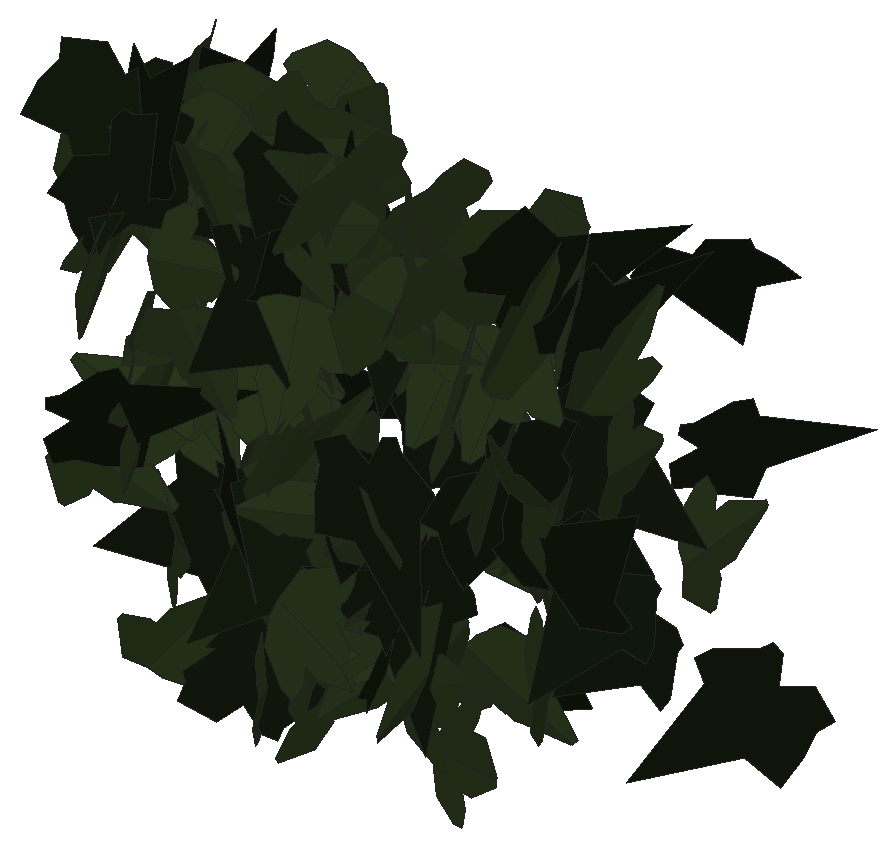
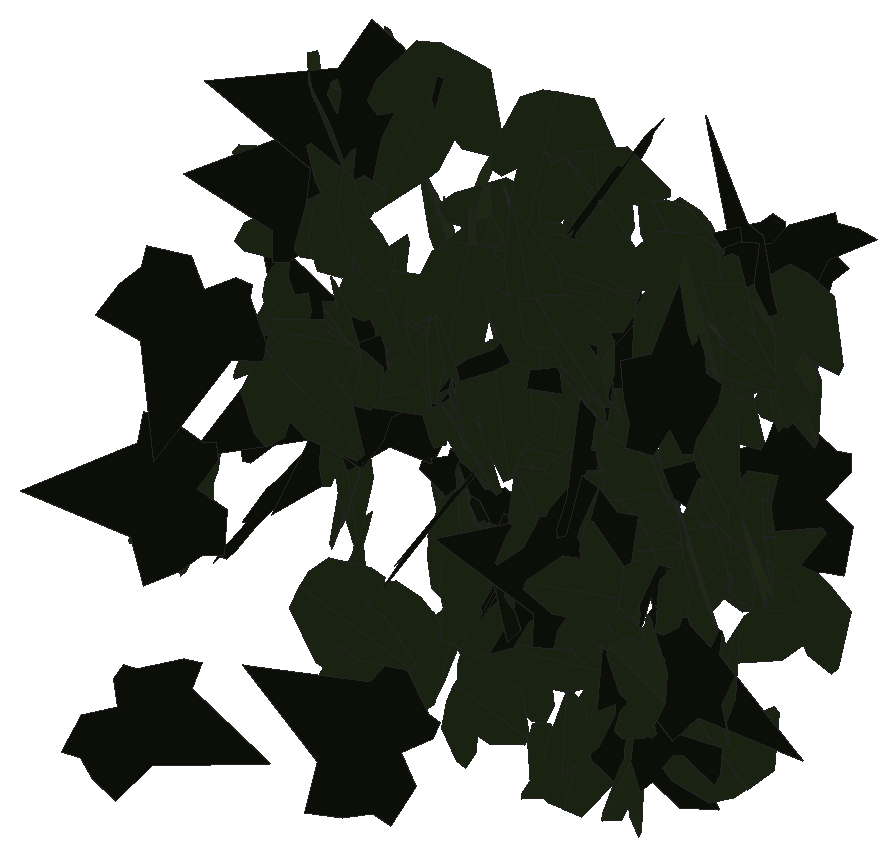
# SketchUp Ruby script. Lengths in inches.
U = 1.inch
M = Sketchup.active_model
def pt(a) = Geom::Point3d.new(a.map { |v| v * U })
def face(e, loops, mat)
  f = e.add_face(loops[0].map { |a| pt(a) })
  loops[1..].each { |l| e.add_face(l.map { |a| pt(a) }).erase! }
  f.material = f.back_material = mat if mat
  f
end
# faces: each face lists its corners as indices into pts; further lists are holes
def faces(e, pts, list, mat = nil) = list.each { |f| face(e, (f[0].is_a?(Array) ? f : [f]).map { |l| l.map { |i| pts[i] } }, mat) }
# xy, xz, yz: faces in a plane at the given z, y or x. An outline is a flat list of corners, or four numbers for a rectangle; further outlines are holes
def ring(l) = l.size == 4 ? [[l[0], l[1]], [l[2], l[1]], [l[2], l[3]], [l[0], l[3]]] : l.each_slice(2).to_a
def flat(e, list, mat, &to3) = list.each { |f| face(e, (f[0].is_a?(Array) ? f : [f]).map { |l| ring(l).map { |u, v| to3.(u, v) } }, mat) }
def xy(e, z, list, mat = nil) = flat(e, list, mat) { |x, y| [x, y, z] }
def xz(e, y, list, mat = nil) = flat(e, list, mat) { |x, z| [x, y, z] }
def yz(e, x, list, mat = nil) = flat(e, list, mat) { |y, z| [x, y, z] }
def lines(e, pts, list) = list.each { |a, b| e.add_line(pt(pts[a]), pt(pts[b])) }
# prism: a flat outline (further loops are holes) pulled along v
def prism(e, loops, v, mat = nil)
  f = face(e, loops, mat); d = Geom::Vector3d.new(v.map { |x| x * U })
  f.pushpull(f.normal.samedirection?(d) ? d.length : -d.length)
end
def box(e, o, s, mat = nil) = prism(e, [[o, [o[0] + s[0], o[1], o[2]], [o[0] + s[0], o[1] + s[1], o[2]], [o[0], o[1] + s[1], o[2]]]], [0, 0, s[2]], mat)
def at(x, y, z, deg = 0) = Geom::Transformation.translation(pt([x, y, z])) * Geom::Transformation.rotation(ORIGIN, Z_AXIS, deg.degrees)
def axes(o, x, y, z) = Geom::Transformation.new([*x, 0, *y, 0, *z, 0, *pt(o).to_a, 1])
def part(name) = M.definitions.add(name)
# library, detail: a bought-in or finely detailed component or shape, given as its bounding box
def library(name, o, s) = part(name).tap { |d| box(d.entities, o, s) }
def detail(e, o, s) = box(e.add_group.entities, o, s)
def put(e, d, t, mat = nil) = e.add_instance(d, t).tap { |i| i.material = mat if mat }
def group(e, t, mat = nil) = e.add_group.tap { |g| g.transformation = t; g.material = mat if mat }.entities
root = M.entities
M.materials.add("efeu1").color = [18, 25, 13]
M.materials.add("efeu2").color = [43, 57, 29]
c1 = part("ivyleaf_10")
p = [[0,0.5,-0.03],[-0.0625,2.02,-0.43],[-0.19,2.01,-0.46],[-0.54,1.05,-0.29],[-0.52,0.625,-0.18],[-0.83,0.76,-0.28],
  [-1.16,0.64,-0.33],[-1.15,0.33,-0.24],[-0.77,-0.39,0.02],[-0.3,-0.51,0.16],[0.04,-0.48,0.23],[-0.02,2.01,-0.4375],
  [-0.06,2.01,-0.43],[0.04,-0.49,0.23],[0.67,-0.49,0.14],[1.38,0.36,-0.2],[1.375,0.51,-0.24],[0.81,0.65,-0.19],
  [0.62,0.59,-0.15],[0.6,1.09,-0.28],[0.5,1.23,-0.31]]
faces(c1.entities,p,[[0,1,2,3,4,5,6,7,8,9,10],[11,12,0,13,14,15,16,17,18,19,20]],"efeu2")
c2 = part("ivyleaf_9")
p = [[1.54,2.16,1.25],[1.36,2.04,1.19],[-0.21,0.99,0.68],[-0.71,1.11,0.82],[-0.85,0.86,0.67],[-0.8,0.17,0.21],
  [-0.9,-0.01,0.1],[-0.67,-0.16,-0.02],[-0.08,-0.08,-0.05],[-0.03,-0.6,-0.4],[0.65,-0.88,-0.66],[0.83,-0.6,-0.49],
  [1.29,-0.42,-0.43],[1.8125,-0.07,-0.26],[1.21,0.44,0.15]]
faces(c2.entities,p,[[0,1,2,3,4,5,6,7,8,9,10,11,12,13,14]],"efeu1")
put(root,c1,axes([531.59,135.63,168.51],[-0.39651,0.03608,0.65448],[0.62652,-0.20395,0.39082],[0.19265,0.73754,0.07605]))
put(root,c1,axes([530.57,135.38,169.3],[0.4498,-0.67197,0.0682],[-0.028,0.06332,0.80854],[-0.67485,-0.45052,0.01191]))
put(root,c1,axes([524.71,135.68,170.1875],[0.13317,-0.67555,0.22901],[0.09772,-0.21349,-0.6866],[0.70659,0.15685,0.0518]))
put(root,c1,axes([529.39,135.33,167.53],[-0.4084,0.02461,0.55664],[-0.55643,0.01796,-0.40903],[-0.02905,-0.69016,0.00921]))
put(root,c2,axes([529.11,135.65,168.17],[0.29259,-0.81264,-0.10232],[-0.03731,0.09532,-0.8637],[0.81821,0.29495,-0.00279]))
put(root,c2,axes([524.8,134.97,167.72],[0.24324,0.53868,-0.57318],[0.23052,0.52479,0.59104],[0.75204,-0.3351,0.00422]))
put(root,c1,axes([528.37,135.0625,165.95],[-0.00344,0.62956,0.46716],[-0.00301,0.46715,-0.62957],[-0.78395,-0.00456,0.00037]))
put(root,c1,axes([528.69,135.78,167.27],[0.00736,0.01589,0.74245],[-0.5731,-0.47205,0.01578],[0.47226,-0.5731,0.00758]))
put(root,c1,axes([530.04,136.0625,165.72],[0.07231,-0.35282,0.70235],[0.17205,-0.6811,-0.35986],[0.76692,0.18606,0.01451]))
put(root,c2,axes([527.125,136.19,169.88],[-0.17709,-0.46496,0.63976],[-0.14722,-0.62476,-0.49481],[0.77705,-0.22433,0.05205]))
put(root,c1,axes([529.74,135.83,165.03],[0.32065,-0.23828,-0.71476],[0.54937,-0.45766,0.39903],[-0.51561,-0.6358,-0.01935]))
put(root,c2,axes([526.64,136.1,166.29],[-0.15856,0.00295,0.8534],[0.08395,-0.86374,0.01858],[0.84927,0.08593,0.15749]))
put(root,c1,axes([531.75,135.19,170.95],[0.26182,-0.59476,0.61403],[-0.20768,0.57869,0.64909],[-0.82924,-0.33272,0.03131]))
put(root,c1,axes([525.67,135.77,170.07],[0.14569,-0.08799,-0.68476],[0.61926,-0.29273,0.16937],[-0.30521,-0.63595,0.01678]))
put(root,c1,axes([530.76,135.37,172.03],[-0.34024,-0.63647,-0.55717],[0.23635,0.50511,-0.72132],[0.8122,-0.41361,-0.0235]))
put(root,c1,axes([527.8,135.91,171.3],[0.23201,-0.23226,-0.7183],[0.65895,-0.30437,0.31126],[-0.36836,-0.69076,0.10437]))
put(root,c2,axes([527.66,136.26,166.49],[-0.52969,-0.47413,0.28475],[-0.20039,-0.20296,-0.71071],[0.51549,-0.56609,0.01632]))
put(root,c1,axes([526.08,135.67,169.24],[-0.68378,-0.15233,-0.18445],[0.1801,0.0398,-0.70054],[0.15744,-0.7071,0.0003]))
put(root,c2,axes([532.01,135.89,167.36],[-0.21716,-0.06392,0.76179],[0.64532,-0.4399,0.14705],[0.40984,0.65877,0.17211]))
put(root,c1,axes([524.65,135.6,169.89],[0.27816,-0.66408,0.30344],[-0.0927,0.28996,0.71957],[-0.72421,-0.29218,0.02444]))
put(root,c1,axes([525.15,136.08,167.83],[0.14834,-0.6526,0.26133],[0.10541,-0.24342,-0.6677],[0.69503,0.1762,0.04549]))
put(root,c1,axes([527.63,135.86,169.73],[0.70962,0.20851,-0.02329],[-0.02405,-0.00075,-0.7396],[-0.20842,0.71,0.00606]))
put(root,c2,axes([525,135.44,171.52],[0.0496,-0.18551,-0.74559],[0.02226,0.74717,-0.18442],[0.76799,-0.00968,0.0535]))
put(root,c2,axes([524.53,136.2,172.16],[-0.29661,-0.7166,-0.13537],[0.06053,0.12144,-0.7755],[0.72676,-0.30258,0.00934]))
put(root,c2,axes([525.02,136.02,171.38],[-0.22619,0.33505,0.65354],[0.26485,-0.60061,0.39958],[0.685,0.34285,0.06131]))
put(root,c2,axes([529.45,136.08,166.65],[-0.50927,-0.22396,-0.63282],[0.58838,0.23345,-0.55613],[0.32314,-0.77802,0.01529]))
put(root,c1,axes([529.29,136.21,165.14],[-0.29206,-0.33727,0.57779],[-0.38365,-0.43207,-0.44612],[0.5481,-0.48214,-0.00439]))
put(root,c1,axes([530.93,135.99,168.77],[0.18073,-0.72055,-0.03775],[-0.00782,0.03696,-0.74287],[0.7215,0.1809,0.0014]))
put(root,c1,axes([526.12,135.89,171.53],[-0.61442,0.2705,-0.22588],[0.20711,-0.09015,-0.67132],[-0.28512,-0.64838,-0.0009]))
put(root,c1,axes([528.6,135.74,172.3],[-0.25568,-0.77369,-0.37196],[0.10203,0.35797,-0.81472],[0.85237,-0.27493,-0.01405]))
put(root,c2,axes([527.33,135.93,172.1875],[0.40346,-0.57241,-0.32294],[-0.16635,0.27766,-0.69997],[0.63583,0.43586,0.02179]))
put(root,c1,axes([527.67,136.01,172.01],[-0.50904,-0.44696,0.07923],[-0.05516,-0.05725,-0.67738],[0.45056,-0.51197,0.00658]))
put(root,c1,axes([524.51,135.91,171.24],[-0.76025,-0.05515,-0.26231],[0.26294,-0.00024,-0.76203],[0.05205,-0.80423,0.01821]))
put(root,c1,axes([524.29,135.81,166.73],[-0.40222,-0.21698,-0.51948],[0.48379,0.19327,-0.45532],[0.28789,-0.62793,0.03937]))
put(root,c1,axes([529.18,135.76,170.67],[-0.39801,-0.32731,-0.64646],[0.55624,0.33466,-0.51191],[0.46437,-0.68141,0.0591]))
put(root,c1,axes([528.95,136.02,165.72],[0.47088,0.11639,0.50683],[0.47941,0.16773,-0.48393],[-0.20147,0.67117,0.03305]))
put(root,c1,axes([525.4,136,163.95],[-0.38309,-0.40564,0.35463],[0.25571,0.24613,0.55776],[-0.47425,0.46037,0.01427]))
put(root,c1,axes([529.36,136.25,165.5],[0.36558,-0.67525,-0.10081],[0.05545,-0.08461,0.76781],[-0.68047,-0.36967,0.00841]))
put(root,c1,axes([528.4375,136.04,165.69],[0.66506,0.16037,-0.13782],[0.13359,0.03394,0.68412],[0.16392,-0.67834,0.00164]))
put(root,c1,axes([527.77,135.76,167.48],[0.09933,-0.44647,0.64173],[-0.08257,0.63728,0.45615],[-0.77739,-0.12473,0.03355]))
put(root,c2,axes([532.29,136.82,167.18],[-0.28597,-0.62776,0.33162],[-0.13912,-0.30103,-0.68983],[0.69621,-0.31801,-0.00163]))
put(root,c1,axes([525.04,136.43,167.14],[0.27394,0.3777,0.53924],[-0.41946,-0.35004,0.45827],[0.50744,-0.49325,0.0877]))
put(root,c1,axes([526.21,136.3,171.96],[0.64179,-0.18739,-0.23723],[-0.22442,0.07766,-0.6685],[0.20255,0.67981,0.01098]))
put(root,c1,axes([531.85,136.53,171.9],[0.54873,-0.47539,0.28764],[0.21523,-0.19085,-0.726],[0.51226,0.58942,-0.00308]))
put(root,c1,axes([525.02,136.57,165.31],[-0.21851,0.12823,0.66954],[0.59328,-0.31054,0.2531],[0.33578,0.63214,-0.01148]))
put(root,c2,axes([527.3,136.54,169.68],[0.4162,0.40639,0.59318],[-0.44093,-0.39714,0.58146],[0.56797,-0.60611,0.01673]))
put(root,c1,axes([528.16,136.59,170.39],[0.24682,-0.40499,-0.55279],[0.39299,-0.39768,0.46682],[-0.56139,-0.45645,0.08375]))
put(root,c1,axes([527.43,135.84,167.23],[0.06635,-0.43948,0.72964],[-0.03839,0.72956,0.44293],[-0.85091,-0.06718,0.03691]))
put(root,c2,axes([529.33,135.88,165.74],[-0.4637,0.24143,-0.6951],[-0.64038,0.27227,0.52177],[0.36243,0.78996,0.0326]))
put(root,c2,axes([526.49,136.31,163.57],[-0.59702,0.09361,0.49924],[0.45949,-0.22888,0.59239],[0.21652,0.74384,0.11945]))
put(root,c1,axes([530.2,135.98,164.11],[-0.13059,0.40394,0.56917],[-0.22728,0.52288,-0.42323],[-0.6599,-0.26002,0.03313]))
put(root,c2,axes([531.18,136.05,171.41],[0.20779,0.0048,0.83066],[0.79376,0.25127,-0.20002],[-0.24488,0.81856,0.05653]))
put(root,c1,axes([527.65,136.875,167.11],[-0.12673,-0.53979,-0.46269],[-0.12428,-0.44593,0.55427],[-0.70001,0.17689,-0.01464]))
put(root,c1,axes([526.96,136.34,164.96],[-0.43065,0.32413,-0.49227],[-0.4355,0.23582,0.53626],[0.39715,0.61006,0.05426]))
put(root,c1,axes([527.15,136.58,169.78],[-0.42261,0.38138,-0.38604],[0.29375,-0.25063,-0.56919],[-0.45628,-0.5146,-0.00888]))
put(root,c1,axes([527.43,136.9,163.45],[-0.13135,-0.56196,-0.43447],[-0.11411,-0.41941,0.57697],[-0.7011,0.17354,-0.0125]))
put(root,c1,axes([529.17,136.53,170.8125],[0.28881,-0.68795,-0.15673],[-0.06917,0.14093,-0.74606],[0.70218,0.29684,-0.00903]))
put(root,c1,axes([529.06,137.07,165.72],[-0.016,0.00559,-0.7466],[-0.29074,-0.68787,0.00108],[-0.68769,0.29069,0.01691]))
put(root,c1,axes([524.93,136.84,171.14],[0.11394,-0.43975,-0.5067],[0.35842,-0.39457,0.42303],[-0.56714,-0.33771,0.16555]))
put(root,c1,axes([529.65,136.08,170.66],[-0.20672,0.40739,-0.74788],[-0.39152,0.63798,0.45575],[0.7563,0.44162,0.03152]))
put(root,c2,axes([528.29,136.24,165.95],[0.64479,0.3981,-0.16174],[-0.14511,-0.07279,-0.75766],[-0.40446,0.66077,0.01398]))
put(root,c1,axes([524.32,136.89,168.23],[0.35167,-0.49671,0.35568],[0.24419,-0.2619,-0.60719],[0.56,0.42613,0.04141]))
put(root,c2,axes([525.94,136.77,165.85],[-0.08076,-0.06061,-0.80323],[-0.65452,-0.4656,0.10094],[-0.46952,0.65947,-0.00256]))
put(root,c1,axes([527.71,137.19,165.3],[-0.12104,-0.29918,0.64305],[0.00431,-0.65265,-0.30283],[0.70923,-0.04709,0.11158]))
put(root,c1,axes([528.6,137.24,164.95],[-0.02881,-0.12579,0.72322],[0.1565,-0.70819,-0.11695],[0.7172,0.14948,0.05457]))
put(root,c2,axes([528.02,136.55,167.23],[0.50992,-0.52739,-0.44858],[-0.29596,0.33762,-0.73336],[0.62593,0.58929,0.0187]))
put(root,c1,axes([527.48,137.09,166.63],[-0.26848,0.27606,0.61112],[0.39362,-0.46807,0.38436],[0.5429,0.47588,0.02354]))
put(root,c1,axes([532.24,136.57,170.12],[0.02248,-0.6388,0.40227],[-0.02157,0.40174,0.63916],[-0.7546,-0.03051,-0.00629]))
put(root,c1,axes([524.96,136.74,167.33],[0.73535,-0.13555,-0.05695],[0.05617,-0.00943,0.74774],[-0.13588,-0.73749,0.0009]))
put(root,c1,axes([530.39,136.91,169.71],[0.73234,0.08478,-0.17386],[-0.17379,-0.01055,-0.73718],[-0.08493,0.75262,0.00925]))
put(root,c1,axes([531.0625,136.76,166.97],[-0.46824,0.5948,-0.09438],[0.0586,-0.07399,-0.75699],[-0.59938,-0.4719,-0.00027]))
put(root,c1,axes([526.71,136.38,163.76],[0,-0.08958,-0.67894],[-0.10214,0.67135,-0.08858],[0.67717,0.10126,-0.01336]))
put(root,c1,axes([524.82,136.46,167.79],[0.0479,0.03506,0.74705],[0.4376,0.60574,-0.05648],[-0.60648,0.43983,0.01824]))
put(root,c1,axes([524.96,136.68,167.5],[0.43714,0.41463,0.44634],[0.3364,0.29372,-0.60232],[-0.50791,0.5514,-0.01479]))
put(root,c2,axes([530.52,136.39,168.28],[0.06665,-0.17459,-0.86218],[-0.15889,0.84804,-0.18401],[0.86521,0.16919,0.03262]))
put(root,c1,axes([531.01,137.07,167.56],[0.08253,-0.74652,-0.09178],[-0.0101,0.09122,-0.75107],[0.75207,0.08315,-0.00001]))
put(root,c2,axes([531.81,136.51,170.61],[0.14369,0.10171,0.75796],[0.55225,0.5197,-0.17443],[-0.52903,0.57014,0.02378]))
put(root,c2,axes([532.02,137.77,166.13],[-0.22867,-0.49886,0.64454],[-0.11692,-0.64243,-0.53871],[0.80662,-0.23454,0.10464]))
put(root,c1,axes([526.83,137.27,169.39],[0.19242,-0.08872,-0.67192],[0.58427,-0.33226,0.21119],[-0.34347,-0.6149,-0.01717]))
put(root,c1,axes([525.06,137.34,171.31],[-0.29675,-0.17989,0.61317],[-0.4839,-0.37828,-0.34517],[0.41734,-0.56652,0.03577]))
put(root,c1,axes([531.16,136.56,165.29],[0.04705,-0.01852,-0.75265],[-0.11577,0.74497,-0.02557],[0.74392,0.1171,0.04362]))
put(root,c1,axes([525.28,137.02,171.93],[-0.6349,-0.34234,-0.28304],[0.24819,0.13607,-0.72131],[0.36839,-0.68169,-0.00184]))
put(root,c1,axes([529.25,137.27,169.43],[0.78052,0.02182,-0.19434],[-0.19417,-0.00855,-0.78082],[-0.02324,0.8043,-0.00303]))
put(root,c1,axes([529.93,137.12,164.96],[-0.52406,-0.02971,-0.53153],[0.53073,0.02912,-0.5249],[0.04159,-0.74587,0.00068]))
put(root,c1,axes([526.29,136.98,168.02],[0.35107,0.35443,0.47626],[0.31495,0.35783,-0.49845],[-0.50324,0.4712,0.02029]))
put(root,c1,axes([532.33,136.74,168.88],[0.03005,-0.21545,-0.73211],[-0.02535,0.73199,-0.21646],[0.76273,0.03282,0.02165]))
put(root,c1,axes([524.83,137.45,172.1],[0.23855,-0.67456,0.04375],[0.01716,-0.04034,-0.71549],[0.67576,0.23915,0.00272]))
put(root,c1,axes([524.32,137.53,169.15],[-0.26782,0.06887,0.65345],[0.63286,-0.16273,0.27653],[0.1767,0.6872,0]))
put(root,c1,axes([525.88,137.21,168.41],[0.23828,0.13975,0.65069],[0.57861,0.298,-0.27588],[-0.32885,0.62559,-0.01394]))
put(root,c1,axes([526.84,137.42,166.54],[0.27694,-0.06751,-0.63438],[-0.62873,0.08832,-0.28387],[0.10812,0.68653,-0.02586]))
put(root,c1,axes([524.46,137.75,167.48],[0.26718,-0.29727,-0.61621],[0.39747,-0.471,0.39955],[-0.55686,-0.47881,-0.01046]))
put(root,c1,axes([530.58,137.95,171.12],[-0.00813,-0.07625,0.70936],[0.25883,-0.66139,-0.06813],[0.66484,0.25656,0.03519]))
put(root,c2,axes([527.83,137.86,170.17],[-0.09918,-0.81121,0.04789],[0.00062,-0.04832,-0.81722],[0.81262,-0.09897,0.00647]))
put(root,c1,axes([528.9375,137.37,169.12],[0.30404,0.05001,0.64634],[0.59768,0.25487,-0.30087],[-0.25108,0.66726,0.06648]))
put(root,c1,axes([528.09,137.5625,169.65],[-0.18828,-0.7134,0.01011],[-0.00078,-0.01025,-0.73783],[0.71348,-0.18827,0.00186]))
put(root,c1,axes([526.12,137.43,167.71],[-0.37733,-0.02111,-0.58524],[0.58515,0.01436,-0.37779],[0.02351,-0.69619,0.00996]))
put(root,c1,axes([525.3,137.8125,169.7],[0.48741,-0.40839,0.33505],[0.24686,-0.22695,-0.63574],[0.46701,0.54619,-0.01364]))
put(root,c1,axes([526.34,137.36,171.42],[-0.13722,-0.08647,0.76358],[0.64711,0.40535,0.16219],[-0.41447,0.6615,0.00042]))
put(root,c1,axes([530.31,137.68,171.15],[0.49998,-0.01298,0.67816],[0.67824,-0.0003,-0.50005],[0.00794,0.84255,0.01028]))
put(root,c1,axes([526.61,137.33,168.05],[-0.37181,0.5281,0.30284],[-0.18071,0.24311,-0.64581],[-0.58133,-0.41333,0.00707]))
put(root,c1,axes([529.01,137.52,168.9],[0.46314,-0.15238,-0.52506],[-0.4653,0.25145,-0.4834],[0.28706,0.65342,0.06358]))
put(root,c2,axes([527.3,137.34,171.07],[-0.2266,0.0833,-0.7197],[-0.7073,0.1379,0.23866],[0.15693,0.74182,0.03645]))
put(root,c2,axes([526.76,137.42,168.29],[-0.016,-0.41579,0.66314],[0.13351,0.6521,0.41209],[-0.77124,0.12151,0.05758]))
put(root,c2,axes([530.84,137.48,168.55],[0.04663,-0.22895,-0.81104],[0.35815,0.74066,-0.18849],[0.76285,-0.33374,0.13808]))
put(root,c2,axes([528.46,137.9375,167.83],[0.43161,-0.65819,-0.2427],[-0.09503,0.22747,-0.78589],[0.69504,0.43983,0.04326]))
put(root,c1,axes([528.44,137.79,171.02],[-0.25161,-0.72302,-0.30589],[0.0974,0.28999,-0.76554],[0.779,-0.26978,-0.00309]))
put(root,c1,axes([529.95,138.33,169.65],[-0.06599,0.10448,-0.70337],[0.44194,-0.54737,-0.12277],[-0.55707,-0.44662,-0.01407]))
put(root,c1,axes([527.79,138.44,165.22],[-0.09379,-0.46555,0.51675],[0.09165,-0.52515,-0.45648],[0.68947,0.00648,0.13097]))
put(root,c1,axes([525.36,137.78,165.87],[0.22979,-0.50666,0.40543],[-0.16241,0.37151,0.55631],[-0.62825,-0.28135,0.00448]))
put(root,c2,axes([524.52,138.39,170.5],[0.19067,0.37002,0.67668],[-0.30444,-0.60434,0.41624],[0.70861,-0.35921,-0.00325]))
put(root,c2,axes([526.06,138.09,167.5],[0.47882,-0.16828,0.62545],[0.60846,-0.14974,-0.50609],[0.22201,0.77333,0.0381]))
put(root,c1,axes([526.82,138.24,170.91],[-0.75397,-0.03287,0.30797],[0.30771,0.01259,0.75469],[-0.03519,0.81435,0.00077]))
put(root,c1,axes([528.57,138.15,170.26],[0.43413,-0.52962,-0.26418],[-0.16605,0.20548,-0.68481],[0.56808,0.4648,0.00172]))
put(root,c1,axes([530.09,138.375,169.51],[0.521,0.25514,0.41856],[0.36007,0.21528,-0.57942],[-0.33262,0.63268,0.02837]))
put(root,c1,axes([530.09,138.62,165.96],[0.32356,0.04676,-0.639],[-0.63812,0.08778,-0.31669],[0.05752,0.71085,0.08114]))
put(root,c1,axes([530.85,138.46,169.23],[-0.28564,0.17518,-0.63915],[-0.56873,0.29249,0.33434],[0.34021,0.63604,0.02229]))
put(root,c2,axes([529.13,138.4,163.95],[0.47139,0.48791,-0.37327],[0.2128,0.31167,0.67615],[0.57628,-0.5142,0.05565]))
put(root,c1,axes([526.18,138.75,171.63],[0.60033,-0.09688,-0.30791],[-0.30561,0.03868,-0.60803],[0.1039,0.67358,-0.00937]))
put(root,c1,axes([526.65,138.49,168.45],[0.06678,0.53267,-0.42449],[-0.00254,0.42672,0.53507],[0.68112,-0.05063,0.04362]))
put(root,c1,axes([525.59,138.57,167.59],[0.11467,-0.34911,0.56753],[-0.03072,0.5725,0.35837],[-0.66561,-0.08657,0.08124]))
put(root,c1,axes([530.1875,139.35,169.6],[-0.37072,-0.33491,0.50786],[-0.38589,-0.33031,-0.49951],[0.4703,-0.53503,-0.00953]))
put(root,c1,axes([532.21,138.6,166.76],[0.08261,-0.01528,-0.72796],[0.14375,0.71855,0.00123],[0.71379,-0.14294,0.084]))
put(root,c1,axes([525.83,138.9,165.18],[0.07169,0.66212,-0.24659],[-0.02854,0.25037,0.66396],[0.70597,-0.05711,0.05189]))
put(root,c2,axes([532.375,140,164.12],[-0.04265,-0.0166,-0.77044],[-0.0709,-0.76827,0.02048],[-0.76735,0.07191,0.04093]))
put(root,c2,axes([531.43,139.56,170.46],[0.50911,0.53705,-0.1811],[-0.12442,-0.1316,-0.74001],[-0.55294,0.52409,-0.00024]))
put(root,c2,axes([531.51,139.6875,167.59],[0.15327,0.46147,-0.58792],[0.20211,0.5522,0.48612],[0.71955,-0.2534,-0.01132]))
